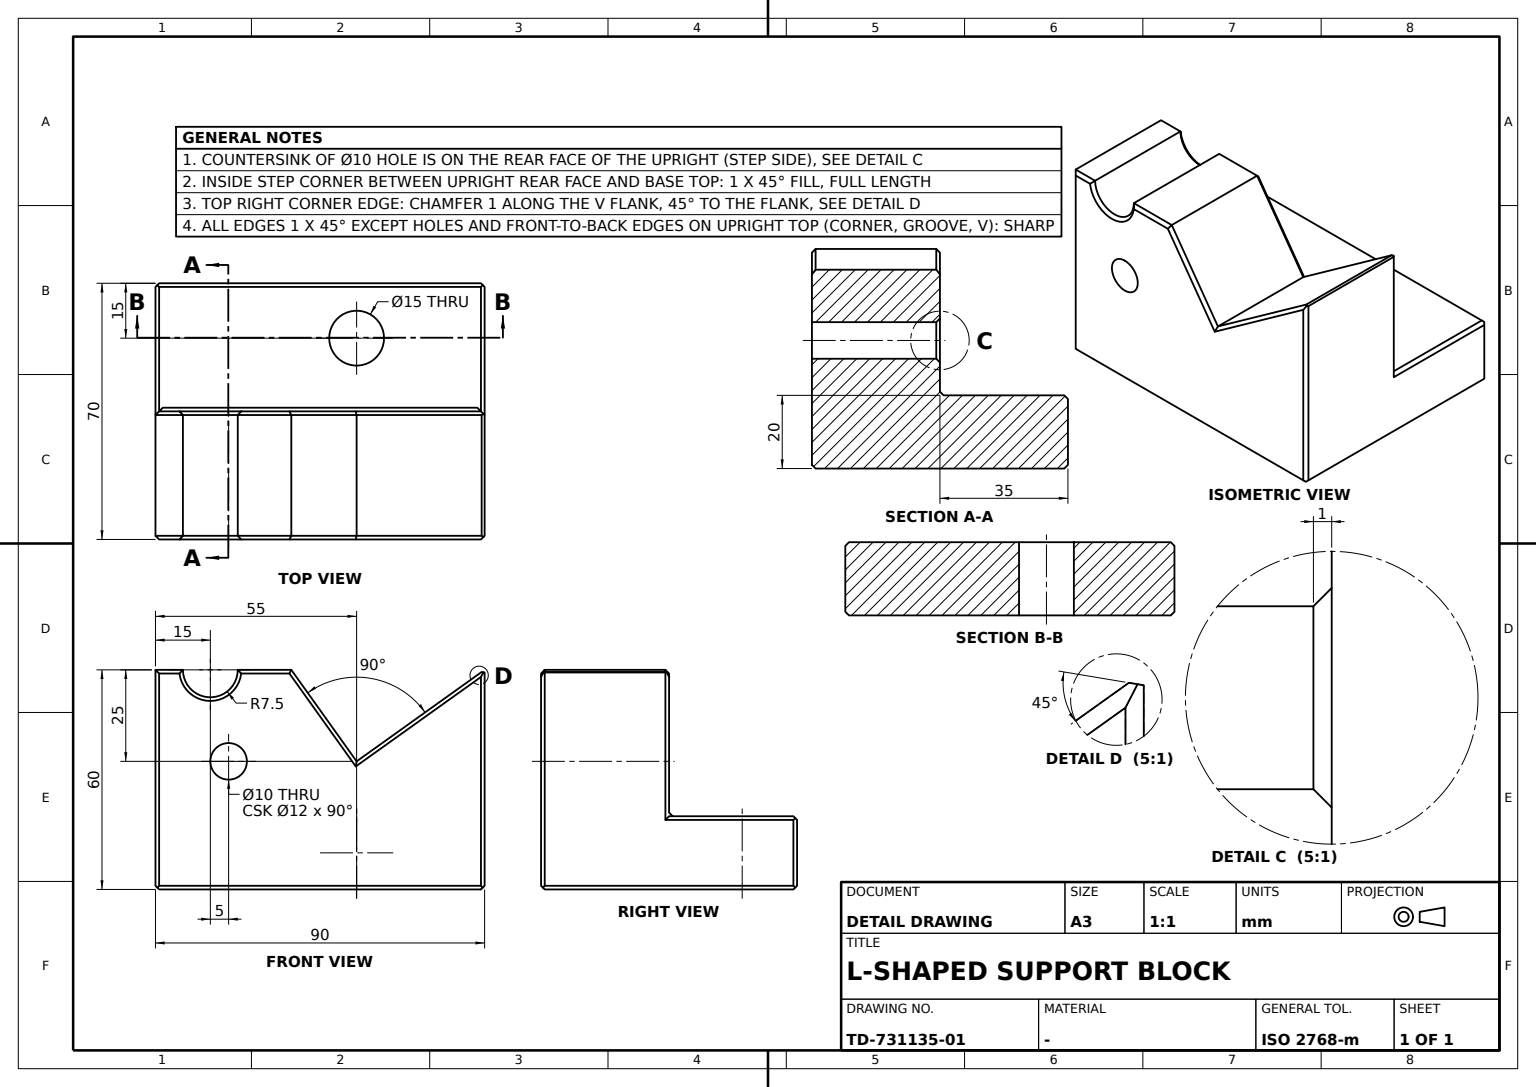
ISO-10303-21;
HEADER;
FILE_DESCRIPTION((''),'2;1');
FILE_NAME('','',(''),(''),'','','');
FILE_SCHEMA(('AUTOMOTIVE_DESIGN'));
ENDSEC;
DATA;
#1=APPLICATION_CONTEXT('');
#2=PRODUCT_CONTEXT('',#1,'mechanical');
#3=PRODUCT('','','',(#2));
#4=PRODUCT_DEFINITION_FORMATION('','',#3);
#5=PRODUCT_DEFINITION_CONTEXT('',#1,'design');
#6=PRODUCT_DEFINITION('','',#4,#5);
#7=PRODUCT_DEFINITION_SHAPE('','',#6);
#8=(LENGTH_UNIT()NAMED_UNIT(*)SI_UNIT(.MILLI.,.METRE.));
#9=(NAMED_UNIT(*)PLANE_ANGLE_UNIT()SI_UNIT($,.RADIAN.));
#10=(NAMED_UNIT(*)SI_UNIT($,.STERADIAN.)SOLID_ANGLE_UNIT());
#11=UNCERTAINTY_MEASURE_WITH_UNIT(LENGTH_MEASURE(0.005),#8,'distance_accuracy_value','');
#12=(GEOMETRIC_REPRESENTATION_CONTEXT(3)GLOBAL_UNCERTAINTY_ASSIGNED_CONTEXT((#11))GLOBAL_UNIT_ASSIGNED_CONTEXT((#8,#9,#10))REPRESENTATION_CONTEXT('',''));
#13=CARTESIAN_POINT('',(-0.813733,-16.5,-0.581238));
#14=VERTEX_POINT('',#13);
#15=CARTESIAN_POINT('',(-0.339767,-16.839767,-0.660233));
#16=VERTEX_POINT('',#15);
#17=CARTESIAN_POINT('',(8.804835,-23.395171,-2.184333));
#18=DIRECTION('',(0.805387266,-0.577350269,-0.134231211));
#19=VECTOR('',#18,1000.);
#20=LINE('',#17,#19);
#21=EDGE_CURVE('',#14,#16,#20,.T.);
#22=ORIENTED_EDGE('',*,*,#21,.F.);
#23=CARTESIAN_POINT('',(-35.,-16.5,-25.));
#24=VERTEX_POINT('',#23);
#25=CARTESIAN_POINT('',(16.018762,-16.5,11.441973));
#26=DIRECTION('',(-0.813733471,0.,-0.581238194));
#27=VECTOR('',#26,1000.);
#28=LINE('',#25,#27);
#29=EDGE_CURVE('',#14,#24,#28,.T.);
#30=ORIENTED_EDGE('',*,*,#29,.T.);
#31=CARTESIAN_POINT('',(-35.232495,-17.5,-26.394972));
#32=VERTEX_POINT('',#31);
#33=CARTESIAN_POINT('',(-39.420834,-35.514728,-51.525007));
#34=DIRECTION('',(-0.134231211,-0.577350269,-0.805387266));
#35=VECTOR('',#34,1000.);
#36=LINE('',#33,#35);
#37=EDGE_CURVE('',#24,#32,#36,.T.);
#38=ORIENTED_EDGE('',*,*,#37,.T.);
#39=CARTESIAN_POINT('',(-1.,-17.5,-1.943189));
#40=VERTEX_POINT('',#39);
#41=CARTESIAN_POINT('',(16.6,-17.5,10.628239));
#42=LINE('',#41,#27);
#43=EDGE_CURVE('',#40,#32,#42,.T.);
#44=ORIENTED_EDGE('',*,*,#43,.F.);
#45=CARTESIAN_POINT('',(6.622712,-9.877288,12.869182));
#46=DIRECTION('',(0.416089715,0.416089715,0.808541092));
#47=VECTOR('',#46,1000.);
#48=LINE('',#45,#47);
#49=EDGE_CURVE('',#40,#16,#48,.T.);
#50=ORIENTED_EDGE('',*,*,#49,.T.);
#51=EDGE_LOOP('',(#22,#30,#38,#44,#50));
#52=FACE_BOUND('',#51,.T.);
#53=DIRECTION('',(-0.410997468,-0.707106781,0.575396456));
#54=AXIS2_PLACEMENT_3D('',#25,#53,#26);
#55=PLANE('',#54);
#56=ADVANCED_FACE('',(#52),#55,.T.);
#57=CARTESIAN_POINT('',(0.,16.5,-41.));
#58=VERTEX_POINT('',#57);
#59=CARTESIAN_POINT('',(0.,51.5,-41.));
#60=VERTEX_POINT('',#59);
#61=CARTESIAN_POINT('',(0.,-31.5,-41.));
#62=DIRECTION('',(0.,1.,0.));
#63=VECTOR('',#62,1000.);
#64=LINE('',#61,#63);
#65=EDGE_CURVE('',#58,#60,#64,.T.);
#66=ORIENTED_EDGE('',*,*,#65,.F.);
#67=CARTESIAN_POINT('',(0.,16.5,-0.71686));
#68=VERTEX_POINT('',#67);
#69=CARTESIAN_POINT('',(0.,16.5,-72.));
#70=DIRECTION('',(0.,0.,-1.));
#71=VECTOR('',#70,1000.);
#72=LINE('',#69,#71);
#73=EDGE_CURVE('',#68,#58,#72,.T.);
#74=ORIENTED_EDGE('',*,*,#73,.F.);
#75=CARTESIAN_POINT('',(0.,-16.5,-0.71686));
#76=VERTEX_POINT('',#75);
#77=CARTESIAN_POINT('',(0.,0.,-0.71686));
#78=LINE('',#77,#63);
#79=EDGE_CURVE('',#76,#68,#78,.T.);
#80=ORIENTED_EDGE('',*,*,#79,.F.);
#81=CARTESIAN_POINT('',(0.,-16.5,-59.));
#82=VERTEX_POINT('',#81);
#83=CARTESIAN_POINT('',(0.,-16.5,0.));
#84=LINE('',#83,#71);
#85=EDGE_CURVE('',#76,#82,#84,.T.);
#86=ORIENTED_EDGE('',*,*,#85,.T.);
#87=CARTESIAN_POINT('',(0.,51.5,-59.));
#88=VERTEX_POINT('',#87);
#89=CARTESIAN_POINT('',(0.,0.,-59.));
#90=LINE('',#89,#63);
#91=EDGE_CURVE('',#82,#88,#90,.T.);
#92=ORIENTED_EDGE('',*,*,#91,.T.);
#93=CARTESIAN_POINT('',(0.,51.5,0.));
#94=DIRECTION('',(0.,0.,1.));
#95=VECTOR('',#94,1000.);
#96=LINE('',#93,#95);
#97=EDGE_CURVE('',#88,#60,#96,.T.);
#98=ORIENTED_EDGE('',*,*,#97,.T.);
#99=EDGE_LOOP('',(#66,#74,#80,#86,#92,#98));
#100=FACE_BOUND('',#99,.T.);
#101=CARTESIAN_POINT('',(0.,0.,0.));
#102=DIRECTION('',(1.,0.,0.));
#103=AXIS2_PLACEMENT_3D('',#101,#102,#62);
#104=PLANE('',#103);
#105=ADVANCED_FACE('',(#100),#104,.T.);
#106=CARTESIAN_POINT('',(-67.5,-16.5,0.));
#107=VERTEX_POINT('',#106);
#108=CARTESIAN_POINT('',(-66.559028,-17.5,-1.));
#109=VERTEX_POINT('',#108);
#110=CARTESIAN_POINT('',(-67.172962,-16.827038,-0.327038));
#111=CARTESIAN_POINT('',(-66.860357,-17.160866,-0.660866));
#112=B_SPLINE_CURVE_WITH_KNOTS('',3,(#106,#110,#111,#108),.UNSPECIFIED.,.F.,.F.,(4,4),(0.,0.001698655),.UNSPECIFIED.);
#113=EDGE_CURVE('',#107,#109,#112,.T.);
#114=ORIENTED_EDGE('',*,*,#113,.T.);
#115=CARTESIAN_POINT('',(-53.371761,-17.5,-1.));
#116=VERTEX_POINT('',#115);
#117=CARTESIAN_POINT('',(-106.6,-17.5,-1.));
#118=VECTOR('',#102,1000.);
#119=LINE('',#117,#118);
#120=EDGE_CURVE('',#109,#116,#119,.T.);
#121=ORIENTED_EDGE('',*,*,#120,.T.);
#122=CARTESIAN_POINT('',(-52.857143,-16.5,0.));
#123=VERTEX_POINT('',#122);
#124=CARTESIAN_POINT('',(-59.14141,-28.71152,-12.21152));
#125=DIRECTION('',(-0.341953402,-0.664480199,-0.664480199));
#126=VECTOR('',#125,1000.);
#127=LINE('',#124,#126);
#128=EDGE_CURVE('',#123,#116,#127,.T.);
#129=ORIENTED_EDGE('',*,*,#128,.F.);
#130=LINE('',#83,#118);
#131=EDGE_CURVE('',#107,#123,#130,.T.);
#132=ORIENTED_EDGE('',*,*,#131,.F.);
#133=EDGE_LOOP('',(#114,#121,#129,#132));
#134=FACE_BOUND('',#133,.T.);
#135=CARTESIAN_POINT('',(-106.6,-16.5,0.));
#136=DIRECTION('',(0.,0.707106781,-0.707106781));
#137=AXIS2_PLACEMENT_3D('',#135,#136,#102);
#138=PLANE('',#137);
#139=ADVANCED_FACE('',(#134),#138,.F.);
#140=CARTESIAN_POINT('',(-1.,17.5,-40.));
#141=VERTEX_POINT('',#140);
#142=CARTESIAN_POINT('',(9.666667,6.833333,-50.666667));
#143=DIRECTION('',(0.577350269,-0.577350269,-0.577350269));
#144=VECTOR('',#143,1000.);
#145=LINE('',#142,#144);
#146=EDGE_CURVE('',#141,#58,#145,.T.);
#147=ORIENTED_EDGE('',*,*,#146,.T.);
#148=ORIENTED_EDGE('',*,*,#65,.T.);
#149=CARTESIAN_POINT('',(-0.5,52.,-40.5));
#150=VERTEX_POINT('',#149);
#151=CARTESIAN_POINT('',(9.666667,41.833333,-50.666667));
#152=LINE('',#151,#144);
#153=EDGE_CURVE('',#150,#60,#152,.T.);
#154=ORIENTED_EDGE('',*,*,#153,.F.);
#155=CARTESIAN_POINT('',(-1.,51.5,-40.));
#156=VERTEX_POINT('',#155);
#157=CARTESIAN_POINT('',(-36.,16.5,-5.));
#158=DIRECTION('',(-0.577350269,-0.577350269,0.577350269));
#159=VECTOR('',#158,1000.);
#160=LINE('',#157,#159);
#161=EDGE_CURVE('',#150,#156,#160,.T.);
#162=ORIENTED_EDGE('',*,*,#161,.T.);
#163=CARTESIAN_POINT('',(-1.,-31.5,-40.));
#164=LINE('',#163,#63);
#165=EDGE_CURVE('',#141,#156,#164,.T.);
#166=ORIENTED_EDGE('',*,*,#165,.F.);
#167=EDGE_LOOP('',(#147,#148,#154,#162,#166));
#168=FACE_BOUND('',#167,.T.);
#169=DIRECTION('',(0.707106781,0.,0.707106781));
#170=AXIS2_PLACEMENT_3D('',#61,#169,#62);
#171=PLANE('',#170);
#172=ADVANCED_FACE('',(#168),#171,.T.);
#173=CARTESIAN_POINT('',(-90.,16.5,0.));
#174=VERTEX_POINT('',#173);
#175=CARTESIAN_POINT('',(-90.,16.5,-41.));
#176=VERTEX_POINT('',#175);
#177=LINE('',#173,#71);
#178=EDGE_CURVE('',#174,#176,#177,.T.);
#179=ORIENTED_EDGE('',*,*,#178,.F.);
#180=CARTESIAN_POINT('',(-89.,17.5,-1.));
#181=VERTEX_POINT('',#180);
#182=CARTESIAN_POINT('',(-65.333333,41.166667,-24.666667));
#183=DIRECTION('',(0.577350269,0.577350269,-0.577350269));
#184=VECTOR('',#183,1000.);
#185=LINE('',#182,#184);
#186=EDGE_CURVE('',#174,#181,#185,.T.);
#187=ORIENTED_EDGE('',*,*,#186,.T.);
#188=CARTESIAN_POINT('',(-89.,17.5,-39.));
#189=VERTEX_POINT('',#188);
#190=CARTESIAN_POINT('',(-89.,17.5,-40.));
#191=LINE('',#190,#95);
#192=EDGE_CURVE('',#189,#181,#191,.T.);
#193=ORIENTED_EDGE('',*,*,#192,.F.);
#194=CARTESIAN_POINT('',(-88.,18.5,-40.));
#195=VERTEX_POINT('',#194);
#196=CARTESIAN_POINT('',(-78.,28.5,-50.));
#197=LINE('',#196,#159);
#198=EDGE_CURVE('',#195,#189,#197,.T.);
#199=ORIENTED_EDGE('',*,*,#198,.F.);
#200=VERTEX_POINT('',#190);
#201=DIRECTION('',(0.707106781,0.707106781,0.));
#202=VECTOR('',#201,1000.);
#203=LINE('',#190,#202);
#204=EDGE_CURVE('',#200,#195,#203,.T.);
#205=ORIENTED_EDGE('',*,*,#204,.F.);
#206=CARTESIAN_POINT('',(-106.,0.5,-57.));
#207=DIRECTION('',(-0.577350269,-0.577350269,-0.577350269));
#208=VECTOR('',#207,1000.);
#209=LINE('',#206,#208);
#210=EDGE_CURVE('',#200,#176,#209,.T.);
#211=ORIENTED_EDGE('',*,*,#210,.T.);
#212=EDGE_LOOP('',(#179,#187,#193,#199,#205,#211));
#213=FACE_BOUND('',#212,.T.);
#214=CARTESIAN_POINT('',(-89.,17.5,-72.));
#215=DIRECTION('',(0.707106781,-0.707106781,0.));
#216=AXIS2_PLACEMENT_3D('',#214,#215,#94);
#217=PLANE('',#216);
#218=ADVANCED_FACE('',(#213),#217,.F.);
#219=CARTESIAN_POINT('',(-82.5,16.5,0.));
#220=VERTEX_POINT('',#219);
#221=CARTESIAN_POINT('',(-83.440972,17.5,-1.));
#222=VERTEX_POINT('',#221);
#223=CARTESIAN_POINT('',(-83.139643,17.160866,-0.660866));
#224=CARTESIAN_POINT('',(-82.827038,16.827038,-0.327038));
#225=B_SPLINE_CURVE_WITH_KNOTS('',3,(#221,#223,#224,#219),.UNSPECIFIED.,.F.,.F.,(4,4),(0.,0.001698655),.UNSPECIFIED.);
#226=EDGE_CURVE('',#220,#222,#225,.F.);
#227=ORIENTED_EDGE('',*,*,#226,.T.);
#228=CARTESIAN_POINT('',(0.,17.5,-1.));
#229=LINE('',#228,#118);
#230=EDGE_CURVE('',#181,#222,#229,.T.);
#231=ORIENTED_EDGE('',*,*,#230,.F.);
#232=ORIENTED_EDGE('',*,*,#186,.F.);
#233=CARTESIAN_POINT('',(-106.6,16.5,0.));
#234=LINE('',#233,#118);
#235=EDGE_CURVE('',#174,#220,#234,.T.);
#236=ORIENTED_EDGE('',*,*,#235,.T.);
#237=EDGE_LOOP('',(#227,#231,#232,#236));
#238=FACE_BOUND('',#237,.T.);
#239=CARTESIAN_POINT('',(-106.6,17.5,-1.));
#240=DIRECTION('',(0.,-0.707106781,-0.707106781));
#241=AXIS2_PLACEMENT_3D('',#239,#240,#102);
#242=PLANE('',#241);
#243=ADVANCED_FACE('',(#238),#242,.F.);
#244=CARTESIAN_POINT('',(-89.,51.5,-40.));
#245=VERTEX_POINT('',#244);
#246=CARTESIAN_POINT('',(-89.,-31.5,-40.));
#247=LINE('',#246,#63);
#248=EDGE_CURVE('',#200,#245,#247,.T.);
#249=ORIENTED_EDGE('',*,*,#248,.T.);
#250=CARTESIAN_POINT('',(-89.5,52.,-40.5));
#251=VERTEX_POINT('',#250);
#252=CARTESIAN_POINT('',(-96.,58.5,-47.));
#253=DIRECTION('',(0.577350269,-0.577350269,0.577350269));
#254=VECTOR('',#253,1000.);
#255=LINE('',#252,#254);
#256=EDGE_CURVE('',#251,#245,#255,.T.);
#257=ORIENTED_EDGE('',*,*,#256,.F.);
#258=CARTESIAN_POINT('',(-90.,51.5,-41.));
#259=VERTEX_POINT('',#258);
#260=CARTESIAN_POINT('',(-117.666667,23.833333,-68.666667));
#261=LINE('',#260,#208);
#262=EDGE_CURVE('',#251,#259,#261,.T.);
#263=ORIENTED_EDGE('',*,*,#262,.T.);
#264=CARTESIAN_POINT('',(-90.,0.,-41.));
#265=LINE('',#264,#63);
#266=EDGE_CURVE('',#176,#259,#265,.T.);
#267=ORIENTED_EDGE('',*,*,#266,.F.);
#268=ORIENTED_EDGE('',*,*,#210,.F.);
#269=EDGE_LOOP('',(#249,#257,#263,#267,#268));
#270=FACE_BOUND('',#269,.T.);
#271=CARTESIAN_POINT('',(-90.,-31.5,-41.));
#272=DIRECTION('',(0.707106781,0.,-0.707106781));
#273=AXIS2_PLACEMENT_3D('',#271,#272,#62);
#274=PLANE('',#273);
#275=ADVANCED_FACE('',(#270),#274,.F.);
#276=CARTESIAN_POINT('',(-90.,-16.5,-59.));
#277=VERTEX_POINT('',#276);
#278=CARTESIAN_POINT('',(-90.,-16.5,0.));
#279=VERTEX_POINT('',#278);
#280=LINE('',#278,#95);
#281=EDGE_CURVE('',#277,#279,#280,.T.);
#282=ORIENTED_EDGE('',*,*,#281,.T.);
#283=CARTESIAN_POINT('',(-90.,17.5,0.));
#284=DIRECTION('',(0.,-1.,0.));
#285=VECTOR('',#284,1000.);
#286=LINE('',#283,#285);
#287=EDGE_CURVE('',#174,#279,#286,.T.);
#288=ORIENTED_EDGE('',*,*,#287,.F.);
#289=ORIENTED_EDGE('',*,*,#178,.T.);
#290=ORIENTED_EDGE('',*,*,#266,.T.);
#291=CARTESIAN_POINT('',(-90.,51.5,-59.));
#292=VERTEX_POINT('',#291);
#293=CARTESIAN_POINT('',(-90.,51.5,0.));
#294=LINE('',#293,#71);
#295=EDGE_CURVE('',#259,#292,#294,.T.);
#296=ORIENTED_EDGE('',*,*,#295,.T.);
#297=CARTESIAN_POINT('',(-90.,0.,-59.));
#298=LINE('',#297,#285);
#299=EDGE_CURVE('',#292,#277,#298,.T.);
#300=ORIENTED_EDGE('',*,*,#299,.T.);
#301=EDGE_LOOP('',(#282,#288,#289,#290,#296,#300));
#302=FACE_BOUND('',#301,.T.);
#303=CARTESIAN_POINT('',(-90.,0.,0.));
#304=AXIS2_PLACEMENT_3D('',#303,#102,#62);
#305=PLANE('',#304);
#306=ADVANCED_FACE('',(#302),#305,.F.);
#307=CARTESIAN_POINT('',(-35.,16.5,-25.));
#308=VERTEX_POINT('',#307);
#309=CARTESIAN_POINT('',(-35.,17.5,-25.));
#310=LINE('',#309,#285);
#311=EDGE_CURVE('',#308,#24,#310,.T.);
#312=ORIENTED_EDGE('',*,*,#311,.F.);
#313=CARTESIAN_POINT('',(-52.857143,16.5,0.));
#314=VERTEX_POINT('',#313);
#315=DIRECTION('',(-0.581238194,0.,0.813733471));
#316=VECTOR('',#315,1000.);
#317=LINE('',#307,#316);
#318=EDGE_CURVE('',#308,#314,#317,.T.);
#319=ORIENTED_EDGE('',*,*,#318,.T.);
#320=CARTESIAN_POINT('',(-52.857143,17.5,0.));
#321=LINE('',#320,#285);
#322=EDGE_CURVE('',#314,#123,#321,.T.);
#323=ORIENTED_EDGE('',*,*,#322,.T.);
#324=CARTESIAN_POINT('',(-1.843742,-16.5,-71.418762));
#325=LINE('',#324,#316);
#326=EDGE_CURVE('',#24,#123,#325,.T.);
#327=ORIENTED_EDGE('',*,*,#326,.F.);
#328=EDGE_LOOP('',(#312,#319,#323,#327));
#329=FACE_BOUND('',#328,.T.);
#330=DIRECTION('',(0.813733471,0.,0.581238194));
#331=AXIS2_PLACEMENT_3D('',#309,#330,#315);
#332=PLANE('',#331);
#333=ADVANCED_FACE('',(#329),#332,.T.);
#334=CARTESIAN_POINT('',(-35.232495,17.5,-26.394972));
#335=VERTEX_POINT('',#334);
#336=CARTESIAN_POINT('',(-37.175831,25.858604,-38.054988));
#337=DIRECTION('',(0.134231211,-0.577350269,0.805387266));
#338=VECTOR('',#337,1000.);
#339=LINE('',#336,#338);
#340=EDGE_CURVE('',#335,#308,#339,.T.);
#341=ORIENTED_EDGE('',*,*,#340,.F.);
#342=CARTESIAN_POINT('',(-53.371761,17.5,-1.));
#343=VERTEX_POINT('',#342);
#344=CARTESIAN_POINT('',(-16.894815,17.5,-52.067725));
#345=LINE('',#344,#316);
#346=EDGE_CURVE('',#335,#343,#345,.T.);
#347=ORIENTED_EDGE('',*,*,#346,.T.);
#348=CARTESIAN_POINT('',(-59.595852,29.594588,-13.094588));
#349=DIRECTION('',(0.341953402,-0.664480199,0.664480199));
#350=VECTOR('',#349,1000.);
#351=LINE('',#348,#350);
#352=EDGE_CURVE('',#343,#314,#351,.T.);
#353=ORIENTED_EDGE('',*,*,#352,.T.);
#354=ORIENTED_EDGE('',*,*,#318,.F.);
#355=EDGE_LOOP('',(#341,#347,#353,#354));
#356=FACE_BOUND('',#355,.T.);
#357=CARTESIAN_POINT('',(-20.657475,17.5,-46.8));
#358=DIRECTION('',(0.575396456,0.707106781,0.410997468));
#359=AXIS2_PLACEMENT_3D('',#357,#358,#315);
#360=PLANE('',#359);
#361=ADVANCED_FACE('',(#356),#360,.T.);
#362=ORIENTED_EDGE('',*,*,#299,.F.);
#363=CARTESIAN_POINT('',(-89.5,52.,-59.5));
#364=VERTEX_POINT('',#363);
#365=CARTESIAN_POINT('',(-113.666667,27.833333,-35.333333));
#366=LINE('',#365,#159);
#367=EDGE_CURVE('',#364,#292,#366,.T.);
#368=ORIENTED_EDGE('',*,*,#367,.F.);
#369=CARTESIAN_POINT('',(-89.,51.5,-60.));
#370=VERTEX_POINT('',#369);
#371=CARTESIAN_POINT('',(-94.266667,56.766667,-54.733333));
#372=LINE('',#371,#144);
#373=EDGE_CURVE('',#364,#370,#372,.T.);
#374=ORIENTED_EDGE('',*,*,#373,.T.);
#375=CARTESIAN_POINT('',(-89.,-16.5,-60.));
#376=VERTEX_POINT('',#375);
#377=CARTESIAN_POINT('',(-89.,65.3,-60.));
#378=LINE('',#377,#285);
#379=EDGE_CURVE('',#370,#376,#378,.T.);
#380=ORIENTED_EDGE('',*,*,#379,.T.);
#381=CARTESIAN_POINT('',(-89.5,-17.,-59.5));
#382=VERTEX_POINT('',#381);
#383=CARTESIAN_POINT('',(-53.8,18.7,-95.2));
#384=LINE('',#383,#184);
#385=EDGE_CURVE('',#382,#376,#384,.T.);
#386=ORIENTED_EDGE('',*,*,#385,.F.);
#387=CARTESIAN_POINT('',(-85.666667,-20.833333,-63.333333));
#388=LINE('',#387,#144);
#389=EDGE_CURVE('',#277,#382,#388,.T.);
#390=ORIENTED_EDGE('',*,*,#389,.F.);
#391=EDGE_LOOP('',(#362,#368,#374,#380,#386,#390));
#392=FACE_BOUND('',#391,.T.);
#393=CARTESIAN_POINT('',(-90.,65.3,-59.));
#394=AXIS2_PLACEMENT_3D('',#393,#169,#284);
#395=PLANE('',#394);
#396=ADVANCED_FACE('',(#392),#395,.F.);
#397=CARTESIAN_POINT('',(-7.71107,-24.21107,0.568318));
#398=DIRECTION('',(-0.702246883,-0.702246883,0.117041147));
#399=VECTOR('',#398,1000.);
#400=LINE('',#397,#399);
#401=EDGE_CURVE('',#76,#16,#400,.T.);
#402=ORIENTED_EDGE('',*,*,#401,.T.);
#403=ORIENTED_EDGE('',*,*,#49,.F.);
#404=CARTESIAN_POINT('',(-1.,-17.5,-59.));
#405=VERTEX_POINT('',#404);
#406=CARTESIAN_POINT('',(-1.,-17.5,0.));
#407=LINE('',#406,#71);
#408=EDGE_CURVE('',#40,#405,#407,.T.);
#409=ORIENTED_EDGE('',*,*,#408,.T.);
#410=CARTESIAN_POINT('',(-0.5,-17.,-59.5));
#411=VERTEX_POINT('',#410);
#412=CARTESIAN_POINT('',(-24.666667,-41.166667,-35.333333));
#413=LINE('',#412,#159);
#414=EDGE_CURVE('',#411,#405,#413,.T.);
#415=ORIENTED_EDGE('',*,*,#414,.F.);
#416=CARTESIAN_POINT('',(23.,6.5,-36.));
#417=DIRECTION('',(0.577350269,0.577350269,0.577350269));
#418=VECTOR('',#417,1000.);
#419=LINE('',#416,#418);
#420=EDGE_CURVE('',#411,#82,#419,.T.);
#421=ORIENTED_EDGE('',*,*,#420,.T.);
#422=ORIENTED_EDGE('',*,*,#85,.F.);
#423=EDGE_LOOP('',(#402,#403,#409,#415,#421,#422));
#424=FACE_BOUND('',#423,.T.);
#425=CARTESIAN_POINT('',(-1.,-17.5,12.));
#426=AXIS2_PLACEMENT_3D('',#425,#215,#70);
#427=PLANE('',#426);
#428=ADVANCED_FACE('',(#424),#427,.T.);
#429=CARTESIAN_POINT('',(-70.,-17.5,-20.));
#430=VERTEX_POINT('',#429);
#431=CARTESIAN_POINT('',(-70.,-17.5,-25.));
#432=AXIS2_PLACEMENT_3D('',#431,#62,#94);
#433=CIRCLE('',#432,5.);
#434=EDGE_CURVE('',#430,#430,#433,.T.);
#435=ORIENTED_EDGE('',*,*,#434,.T.);
#436=EDGE_LOOP('',(#435));
#437=FACE_BOUND('',#436,.T.);
#438=ORIENTED_EDGE('',*,*,#408,.F.);
#439=ORIENTED_EDGE('',*,*,#43,.T.);
#440=CARTESIAN_POINT('',(-2.657475,-17.5,-72.));
#441=LINE('',#440,#316);
#442=EDGE_CURVE('',#32,#116,#441,.T.);
#443=ORIENTED_EDGE('',*,*,#442,.T.);
#444=ORIENTED_EDGE('',*,*,#120,.F.);
#445=CARTESIAN_POINT('',(-83.440972,-17.5,-1.));
#446=VERTEX_POINT('',#445);
#447=CARTESIAN_POINT('',(-75.,-17.5,0.));
#448=AXIS2_PLACEMENT_3D('',#447,#62,#94);
#449=CIRCLE('',#448,8.5);
#450=EDGE_CURVE('',#109,#446,#449,.T.);
#451=ORIENTED_EDGE('',*,*,#450,.T.);
#452=CARTESIAN_POINT('',(-89.,-17.5,-1.));
#453=VERTEX_POINT('',#452);
#454=EDGE_CURVE('',#453,#446,#119,.T.);
#455=ORIENTED_EDGE('',*,*,#454,.F.);
#456=CARTESIAN_POINT('',(-89.,-17.5,-59.));
#457=VERTEX_POINT('',#456);
#458=CARTESIAN_POINT('',(-89.,-17.5,-72.));
#459=LINE('',#458,#95);
#460=EDGE_CURVE('',#457,#453,#459,.T.);
#461=ORIENTED_EDGE('',*,*,#460,.F.);
#462=CARTESIAN_POINT('',(16.6,-17.5,-59.));
#463=DIRECTION('',(-1.,0.,0.));
#464=VECTOR('',#463,1000.);
#465=LINE('',#462,#464);
#466=EDGE_CURVE('',#405,#457,#465,.T.);
#467=ORIENTED_EDGE('',*,*,#466,.F.);
#468=EDGE_LOOP('',(#438,#439,#443,#444,#451,#455,#461,#467));
#469=FACE_BOUND('',#468,.T.);
#470=CARTESIAN_POINT('',(0.,-17.5,0.));
#471=AXIS2_PLACEMENT_3D('',#470,#62,#70);
#472=PLANE('',#471);
#473=ADVANCED_FACE('',(#437,#469),#472,.F.);
#474=ORIENTED_EDGE('',*,*,#460,.T.);
#475=CARTESIAN_POINT('',(-95.533333,-10.966667,5.533333));
#476=LINE('',#475,#144);
#477=EDGE_CURVE('',#279,#453,#476,.T.);
#478=ORIENTED_EDGE('',*,*,#477,.F.);
#479=ORIENTED_EDGE('',*,*,#281,.F.);
#480=ORIENTED_EDGE('',*,*,#389,.T.);
#481=CARTESIAN_POINT('',(-94.,-12.5,-64.));
#482=LINE('',#481,#254);
#483=EDGE_CURVE('',#382,#457,#482,.T.);
#484=ORIENTED_EDGE('',*,*,#483,.T.);
#485=EDGE_LOOP('',(#474,#478,#479,#480,#484));
#486=FACE_BOUND('',#485,.T.);
#487=CARTESIAN_POINT('',(-90.,-16.5,-72.));
#488=AXIS2_PLACEMENT_3D('',#487,#201,#94);
#489=PLANE('',#488);
#490=ADVANCED_FACE('',(#486),#489,.F.);
#491=CARTESIAN_POINT('',(-2.,18.5,-40.));
#492=VERTEX_POINT('',#491);
#493=CARTESIAN_POINT('',(0.,18.5,-40.));
#494=LINE('',#493,#118);
#495=EDGE_CURVE('',#195,#492,#494,.T.);
#496=ORIENTED_EDGE('',*,*,#495,.F.);
#497=ORIENTED_EDGE('',*,*,#198,.T.);
#498=CARTESIAN_POINT('',(-1.,17.5,-39.));
#499=VERTEX_POINT('',#498);
#500=CARTESIAN_POINT('',(-108.,17.5,-39.));
#501=LINE('',#500,#118);
#502=EDGE_CURVE('',#189,#499,#501,.T.);
#503=ORIENTED_EDGE('',*,*,#502,.T.);
#504=CARTESIAN_POINT('',(-12.,28.5,-50.));
#505=LINE('',#504,#254);
#506=EDGE_CURVE('',#492,#499,#505,.T.);
#507=ORIENTED_EDGE('',*,*,#506,.F.);
#508=EDGE_LOOP('',(#496,#497,#503,#507));
#509=FACE_BOUND('',#508,.T.);
#510=DIRECTION('',(0.,0.707106781,0.707106781));
#511=AXIS2_PLACEMENT_3D('',#500,#510,#102);
#512=PLANE('',#511);
#513=ADVANCED_FACE('',(#509),#512,.T.);
#514=ORIENTED_EDGE('',*,*,#434,.F.);
#515=EDGE_LOOP('',(#514));
#516=FACE_BOUND('',#515,.T.);
#517=CARTESIAN_POINT('',(-70.,16.5,-20.));
#518=VERTEX_POINT('',#517);
#519=CARTESIAN_POINT('',(-70.,16.5,-25.));
#520=AXIS2_PLACEMENT_3D('',#519,#62,#94);
#521=CIRCLE('',#520,5.);
#522=EDGE_CURVE('',#518,#518,#521,.F.);
#523=ORIENTED_EDGE('',*,*,#522,.F.);
#524=EDGE_LOOP('',(#523));
#525=FACE_BOUND('',#524,.T.);
#526=CARTESIAN_POINT('',(-70.,-0.66,-25.));
#527=AXIS2_PLACEMENT_3D('',#526,#62,#463);
#528=CYLINDRICAL_SURFACE('',#527,5.);
#529=ADVANCED_FACE('',(#516,#525),#528,.F.);
#530=ORIENTED_EDGE('',*,*,#352,.F.);
#531=CARTESIAN_POINT('',(-66.559028,17.5,-1.));
#532=VERTEX_POINT('',#531);
#533=EDGE_CURVE('',#532,#343,#229,.T.);
#534=ORIENTED_EDGE('',*,*,#533,.F.);
#535=CARTESIAN_POINT('',(-67.5,16.5,0.));
#536=VERTEX_POINT('',#535);
#537=CARTESIAN_POINT('',(-66.860357,17.160866,-0.660866));
#538=CARTESIAN_POINT('',(-67.172962,16.827038,-0.327038));
#539=B_SPLINE_CURVE_WITH_KNOTS('',3,(#531,#537,#538,#535),.UNSPECIFIED.,.F.,.F.,(4,4),(0.,0.001698655),.UNSPECIFIED.);
#540=EDGE_CURVE('',#532,#536,#539,.T.);
#541=ORIENTED_EDGE('',*,*,#540,.T.);
#542=EDGE_CURVE('',#536,#314,#234,.T.);
#543=ORIENTED_EDGE('',*,*,#542,.T.);
#544=EDGE_LOOP('',(#530,#534,#541,#543));
#545=FACE_BOUND('',#544,.T.);
#546=ADVANCED_FACE('',(#545),#242,.F.);
#547=CARTESIAN_POINT('',(-42.5,37.5,-40.));
#548=VERTEX_POINT('',#547);
#549=CARTESIAN_POINT('',(-35.,37.5,-40.));
#550=AXIS2_PLACEMENT_3D('',#549,#70,#463);
#551=CIRCLE('',#550,7.5);
#552=EDGE_CURVE('',#548,#548,#551,.F.);
#553=ORIENTED_EDGE('',*,*,#552,.F.);
#554=EDGE_LOOP('',(#553));
#555=FACE_BOUND('',#554,.T.);
#556=CARTESIAN_POINT('',(-108.,51.5,-40.));
#557=LINE('',#556,#118);
#558=EDGE_CURVE('',#245,#156,#557,.T.);
#559=ORIENTED_EDGE('',*,*,#558,.F.);
#560=ORIENTED_EDGE('',*,*,#248,.F.);
#561=ORIENTED_EDGE('',*,*,#204,.T.);
#562=ORIENTED_EDGE('',*,*,#495,.T.);
#563=DIRECTION('',(-0.707106781,0.707106781,0.));
#564=VECTOR('',#563,1000.);
#565=LINE('',#140,#564);
#566=EDGE_CURVE('',#141,#492,#565,.T.);
#567=ORIENTED_EDGE('',*,*,#566,.F.);
#568=ORIENTED_EDGE('',*,*,#165,.T.);
#569=EDGE_LOOP('',(#559,#560,#561,#562,#567,#568));
#570=FACE_BOUND('',#569,.T.);
#571=CARTESIAN_POINT('',(0.,52.5,-40.));
#572=AXIS2_PLACEMENT_3D('',#571,#70,#284);
#573=PLANE('',#572);
#574=ADVANCED_FACE('',(#555,#570),#573,.F.);
#575=CARTESIAN_POINT('',(-0.5,52.,-59.5));
#576=VERTEX_POINT('',#575);
#577=CARTESIAN_POINT('',(27.,24.5,-32.));
#578=LINE('',#577,#254);
#579=EDGE_CURVE('',#576,#88,#578,.T.);
#580=ORIENTED_EDGE('',*,*,#579,.F.);
#581=CARTESIAN_POINT('',(-1.,52.5,-59.));
#582=VERTEX_POINT('',#581);
#583=CARTESIAN_POINT('',(-35.933333,87.433333,-24.066667));
#584=DIRECTION('',(-0.577350269,0.577350269,0.577350269));
#585=VECTOR('',#584,1000.);
#586=LINE('',#583,#585);
#587=EDGE_CURVE('',#576,#582,#586,.T.);
#588=ORIENTED_EDGE('',*,*,#587,.T.);
#589=CARTESIAN_POINT('',(-1.,52.5,-41.));
#590=VERTEX_POINT('',#589);
#591=CARTESIAN_POINT('',(-1.,52.5,-60.));
#592=LINE('',#591,#95);
#593=EDGE_CURVE('',#582,#590,#592,.T.);
#594=ORIENTED_EDGE('',*,*,#593,.T.);
#595=CARTESIAN_POINT('',(-11.333333,62.833333,-51.333333));
#596=DIRECTION('',(-0.577350269,0.577350269,-0.577350269));
#597=VECTOR('',#596,1000.);
#598=LINE('',#595,#597);
#599=EDGE_CURVE('',#150,#590,#598,.T.);
#600=ORIENTED_EDGE('',*,*,#599,.F.);
#601=ORIENTED_EDGE('',*,*,#153,.T.);
#602=ORIENTED_EDGE('',*,*,#97,.F.);
#603=EDGE_LOOP('',(#580,#588,#594,#600,#601,#602));
#604=FACE_BOUND('',#603,.T.);
#605=CARTESIAN_POINT('',(-1.,52.5,-72.));
#606=AXIS2_PLACEMENT_3D('',#605,#201,#94);
#607=PLANE('',#606);
#608=ADVANCED_FACE('',(#604),#607,.T.);
#609=ORIENTED_EDGE('',*,*,#414,.T.);
#610=ORIENTED_EDGE('',*,*,#466,.T.);
#611=ORIENTED_EDGE('',*,*,#483,.F.);
#612=ORIENTED_EDGE('',*,*,#385,.T.);
#613=CARTESIAN_POINT('',(-1.,-16.5,-60.));
#614=VERTEX_POINT('',#613);
#615=CARTESIAN_POINT('',(0.,-16.5,-60.));
#616=LINE('',#615,#464);
#617=EDGE_CURVE('',#614,#376,#616,.T.);
#618=ORIENTED_EDGE('',*,*,#617,.F.);
#619=CARTESIAN_POINT('',(4.866667,-22.366667,-54.133333));
#620=LINE('',#619,#597);
#621=EDGE_CURVE('',#411,#614,#620,.T.);
#622=ORIENTED_EDGE('',*,*,#621,.F.);
#623=EDGE_LOOP('',(#609,#610,#611,#612,#618,#622));
#624=FACE_BOUND('',#623,.T.);
#625=CARTESIAN_POINT('',(16.6,-16.5,-60.));
#626=AXIS2_PLACEMENT_3D('',#625,#510,#463);
#627=PLANE('',#626);
#628=ADVANCED_FACE('',(#624),#627,.F.);
#629=ORIENTED_EDGE('',*,*,#340,.T.);
#630=CARTESIAN_POINT('',(-0.813733,16.5,-0.581238));
#631=VERTEX_POINT('',#630);
#632=CARTESIAN_POINT('',(0.,16.5,0.));
#633=LINE('',#632,#27);
#634=EDGE_CURVE('',#631,#308,#633,.T.);
#635=ORIENTED_EDGE('',*,*,#634,.F.);
#636=CARTESIAN_POINT('',(-0.339767,16.839767,-0.660233));
#637=VERTEX_POINT('',#636);
#638=CARTESIAN_POINT('',(-23.040282,0.566667,3.123187));
#639=DIRECTION('',(0.805387266,0.577350269,-0.134231211));
#640=VECTOR('',#639,1000.);
#641=LINE('',#638,#640);
#642=EDGE_CURVE('',#631,#637,#641,.T.);
#643=ORIENTED_EDGE('',*,*,#642,.T.);
#644=CARTESIAN_POINT('',(-1.,17.5,-1.943189));
#645=VERTEX_POINT('',#644);
#646=CARTESIAN_POINT('',(4.639441,11.860559,9.015313));
#647=DIRECTION('',(-0.416089715,0.416089715,-0.808541092));
#648=VECTOR('',#647,1000.);
#649=LINE('',#646,#648);
#650=EDGE_CURVE('',#637,#645,#649,.T.);
#651=ORIENTED_EDGE('',*,*,#650,.T.);
#652=CARTESIAN_POINT('',(-18.337681,17.5,-14.327247));
#653=LINE('',#652,#27);
#654=EDGE_CURVE('',#645,#335,#653,.T.);
#655=ORIENTED_EDGE('',*,*,#654,.T.);
#656=EDGE_LOOP('',(#629,#635,#643,#651,#655));
#657=FACE_BOUND('',#656,.T.);
#658=CARTESIAN_POINT('',(12.640465,17.5,7.8));
#659=DIRECTION('',(-0.410997468,0.707106781,0.575396456));
#660=AXIS2_PLACEMENT_3D('',#658,#659,#26);
#661=PLANE('',#660);
#662=ADVANCED_FACE('',(#657),#661,.T.);
#663=CARTESIAN_POINT('',(-1.,51.5,-60.));
#664=VERTEX_POINT('',#663);
#665=CARTESIAN_POINT('',(-1.,-17.5,-60.));
#666=LINE('',#665,#63);
#667=EDGE_CURVE('',#614,#664,#666,.T.);
#668=ORIENTED_EDGE('',*,*,#667,.F.);
#669=ORIENTED_EDGE('',*,*,#617,.T.);
#670=ORIENTED_EDGE('',*,*,#379,.F.);
#671=CARTESIAN_POINT('',(0.,51.5,-60.));
#672=LINE('',#671,#118);
#673=EDGE_CURVE('',#370,#664,#672,.T.);
#674=ORIENTED_EDGE('',*,*,#673,.T.);
#675=EDGE_LOOP('',(#668,#669,#670,#674));
#676=FACE_BOUND('',#675,.T.);
#677=CARTESIAN_POINT('',(-27.5,37.5,-60.));
#678=VERTEX_POINT('',#677);
#679=CARTESIAN_POINT('',(-35.,37.5,-60.));
#680=AXIS2_PLACEMENT_3D('',#679,#94,#102);
#681=CIRCLE('',#680,7.5);
#682=EDGE_CURVE('',#678,#678,#681,.T.);
#683=ORIENTED_EDGE('',*,*,#682,.T.);
#684=EDGE_LOOP('',(#683));
#685=FACE_BOUND('',#684,.T.);
#686=CARTESIAN_POINT('',(0.,-17.5,-60.));
#687=AXIS2_PLACEMENT_3D('',#686,#94,#62);
#688=PLANE('',#687);
#689=ADVANCED_FACE('',(#676,#685),#688,.F.);
#690=ORIENTED_EDGE('',*,*,#682,.F.);
#691=EDGE_LOOP('',(#690));
#692=FACE_BOUND('',#691,.T.);
#693=ORIENTED_EDGE('',*,*,#552,.T.);
#694=EDGE_LOOP('',(#693));
#695=FACE_BOUND('',#694,.T.);
#696=CARTESIAN_POINT('',(-35.,37.5,-85.));
#697=AXIS2_PLACEMENT_3D('',#696,#94,#102);
#698=CYLINDRICAL_SURFACE('',#697,7.5);
#699=ADVANCED_FACE('',(#692,#695),#698,.F.);
#700=ORIENTED_EDGE('',*,*,#21,.T.);
#701=ORIENTED_EDGE('',*,*,#401,.F.);
#702=ORIENTED_EDGE('',*,*,#79,.T.);
#703=CARTESIAN_POINT('',(4.872587,11.627413,-1.528958));
#704=DIRECTION('',(-0.702246883,0.702246883,0.117041147));
#705=VECTOR('',#704,1000.);
#706=LINE('',#703,#705);
#707=EDGE_CURVE('',#68,#637,#706,.T.);
#708=ORIENTED_EDGE('',*,*,#707,.T.);
#709=ORIENTED_EDGE('',*,*,#642,.F.);
#710=CARTESIAN_POINT('',(-0.813733,-31.3,-0.581238));
#711=LINE('',#710,#63);
#712=EDGE_CURVE('',#14,#631,#711,.T.);
#713=ORIENTED_EDGE('',*,*,#712,.F.);
#714=EDGE_LOOP('',(#700,#701,#702,#708,#709,#713));
#715=FACE_BOUND('',#714,.T.);
#716=DIRECTION('',(-0.164398987,0.,-0.986393924));
#717=AXIS2_PLACEMENT_3D('',#710,#716,#62);
#718=PLANE('',#717);
#719=ADVANCED_FACE('',(#715),#718,.F.);
#720=CARTESIAN_POINT('',(-28.666667,23.833333,-87.666667));
#721=LINE('',#720,#208);
#722=EDGE_CURVE('',#576,#664,#721,.T.);
#723=ORIENTED_EDGE('',*,*,#722,.F.);
#724=ORIENTED_EDGE('',*,*,#579,.T.);
#725=ORIENTED_EDGE('',*,*,#91,.F.);
#726=ORIENTED_EDGE('',*,*,#420,.F.);
#727=ORIENTED_EDGE('',*,*,#621,.T.);
#728=ORIENTED_EDGE('',*,*,#667,.T.);
#729=EDGE_LOOP('',(#723,#724,#725,#726,#727,#728));
#730=FACE_BOUND('',#729,.T.);
#731=CARTESIAN_POINT('',(-1.,-31.5,-60.));
#732=AXIS2_PLACEMENT_3D('',#731,#272,#62);
#733=PLANE('',#732);
#734=ADVANCED_FACE('',(#730),#733,.T.);
#735=CARTESIAN_POINT('',(-75.,16.5,0.));
#736=AXIS2_PLACEMENT_3D('',#735,#62,#94);
#737=CIRCLE('',#736,7.5);
#738=EDGE_CURVE('',#220,#536,#737,.F.);
#739=ORIENTED_EDGE('',*,*,#738,.F.);
#740=CARTESIAN_POINT('',(-82.5,-16.5,0.));
#741=VERTEX_POINT('',#740);
#742=LINE('',#219,#63);
#743=EDGE_CURVE('',#741,#220,#742,.T.);
#744=ORIENTED_EDGE('',*,*,#743,.F.);
#745=CARTESIAN_POINT('',(-75.,-16.5,0.));
#746=AXIS2_PLACEMENT_3D('',#745,#284,#70);
#747=CIRCLE('',#746,7.5);
#748=EDGE_CURVE('',#107,#741,#747,.F.);
#749=ORIENTED_EDGE('',*,*,#748,.F.);
#750=LINE('',#535,#63);
#751=EDGE_CURVE('',#536,#107,#750,.F.);
#752=ORIENTED_EDGE('',*,*,#751,.F.);
#753=EDGE_LOOP('',(#739,#744,#749,#752));
#754=FACE_BOUND('',#753,.T.);
#755=CARTESIAN_POINT('',(-75.,-0.66,0.));
#756=AXIS2_PLACEMENT_3D('',#755,#62,#463);
#757=CYLINDRICAL_SURFACE('',#756,7.5);
#758=ADVANCED_FACE('',(#754),#757,.F.);
#759=ORIENTED_EDGE('',*,*,#128,.T.);
#760=ORIENTED_EDGE('',*,*,#442,.F.);
#761=ORIENTED_EDGE('',*,*,#37,.F.);
#762=ORIENTED_EDGE('',*,*,#326,.T.);
#763=EDGE_LOOP('',(#759,#760,#761,#762));
#764=FACE_BOUND('',#763,.T.);
#765=DIRECTION('',(0.575396456,-0.707106781,0.410997468));
#766=AXIS2_PLACEMENT_3D('',#324,#765,#315);
#767=PLANE('',#766);
#768=ADVANCED_FACE('',(#764),#767,.T.);
#769=CARTESIAN_POINT('',(-70.,17.5,-31.));
#770=VERTEX_POINT('',#769);
#771=CARTESIAN_POINT('',(-70.,17.5,-25.));
#772=AXIS2_PLACEMENT_3D('',#771,#284,#70);
#773=CIRCLE('',#772,6.);
#774=EDGE_CURVE('',#770,#770,#773,.T.);
#775=ORIENTED_EDGE('',*,*,#774,.F.);
#776=EDGE_LOOP('',(#775));
#777=FACE_BOUND('',#776,.T.);
#778=ORIENTED_EDGE('',*,*,#522,.T.);
#779=EDGE_LOOP('',(#778));
#780=FACE_BOUND('',#779,.T.);
#781=CARTESIAN_POINT('',(-70.,11.5,-25.));
#782=DIRECTION('',(-0.865680914,0.,0.5005962));
#783=AXIS2_PLACEMENT_3D('',#781,#62,#782);
#784=CONICAL_SURFACE('',#783,0.,0.785398163);
#785=ADVANCED_FACE('',(#777,#780),#784,.F.);
#786=ORIENTED_EDGE('',*,*,#650,.F.);
#787=ORIENTED_EDGE('',*,*,#707,.F.);
#788=ORIENTED_EDGE('',*,*,#73,.T.);
#789=ORIENTED_EDGE('',*,*,#146,.F.);
#790=ORIENTED_EDGE('',*,*,#566,.T.);
#791=ORIENTED_EDGE('',*,*,#506,.T.);
#792=LINE('',#140,#95);
#793=EDGE_CURVE('',#499,#645,#792,.T.);
#794=ORIENTED_EDGE('',*,*,#793,.T.);
#795=EDGE_LOOP('',(#786,#787,#788,#789,#790,#791,#794));
#796=FACE_BOUND('',#795,.T.);
#797=CARTESIAN_POINT('',(-1.,17.5,-72.));
#798=AXIS2_PLACEMENT_3D('',#797,#201,#94);
#799=PLANE('',#798);
#800=ADVANCED_FACE('',(#796),#799,.T.);
#801=ORIENTED_EDGE('',*,*,#712,.T.);
#802=ORIENTED_EDGE('',*,*,#634,.T.);
#803=ORIENTED_EDGE('',*,*,#311,.T.);
#804=ORIENTED_EDGE('',*,*,#29,.F.);
#805=EDGE_LOOP('',(#801,#802,#803,#804));
#806=FACE_BOUND('',#805,.T.);
#807=CARTESIAN_POINT('',(0.,17.5,0.));
#808=AXIS2_PLACEMENT_3D('',#807,#315,#26);
#809=PLANE('',#808);
#810=ADVANCED_FACE('',(#806),#809,.T.);
#811=CARTESIAN_POINT('',(-75.,17.5,0.));
#812=AXIS2_PLACEMENT_3D('',#811,#284,#70);
#813=CIRCLE('',#812,8.5);
#814=EDGE_CURVE('',#222,#532,#813,.T.);
#815=ORIENTED_EDGE('',*,*,#814,.F.);
#816=ORIENTED_EDGE('',*,*,#226,.F.);
#817=ORIENTED_EDGE('',*,*,#738,.T.);
#818=ORIENTED_EDGE('',*,*,#540,.F.);
#819=EDGE_LOOP('',(#815,#816,#817,#818));
#820=FACE_BOUND('',#819,.T.);
#821=CARTESIAN_POINT('',(-75.,9.,0.));
#822=DIRECTION('',(0.397396371,0.,-0.917647059));
#823=AXIS2_PLACEMENT_3D('',#821,#62,#822);
#824=CONICAL_SURFACE('',#823,0.,0.785398163);
#825=ADVANCED_FACE('',(#820),#824,.F.);
#826=CARTESIAN_POINT('',(-89.,52.5,-59.));
#827=VERTEX_POINT('',#826);
#828=CARTESIAN_POINT('',(-107.8,52.5,-59.));
#829=LINE('',#828,#118);
#830=EDGE_CURVE('',#827,#582,#829,.T.);
#831=ORIENTED_EDGE('',*,*,#830,.F.);
#832=CARTESIAN_POINT('',(-89.,52.5,-41.));
#833=VERTEX_POINT('',#832);
#834=CARTESIAN_POINT('',(-89.,52.5,12.));
#835=LINE('',#834,#71);
#836=EDGE_CURVE('',#833,#827,#835,.T.);
#837=ORIENTED_EDGE('',*,*,#836,.F.);
#838=CARTESIAN_POINT('',(0.,52.5,-41.));
#839=LINE('',#838,#118);
#840=EDGE_CURVE('',#833,#590,#839,.T.);
#841=ORIENTED_EDGE('',*,*,#840,.T.);
#842=ORIENTED_EDGE('',*,*,#593,.F.);
#843=EDGE_LOOP('',(#831,#837,#841,#842));
#844=FACE_BOUND('',#843,.T.);
#845=CARTESIAN_POINT('',(0.,52.5,-60.));
#846=AXIS2_PLACEMENT_3D('',#845,#284,#94);
#847=PLANE('',#846);
#848=ADVANCED_FACE('',(#844),#847,.F.);
#849=ORIENTED_EDGE('',*,*,#367,.T.);
#850=ORIENTED_EDGE('',*,*,#295,.F.);
#851=ORIENTED_EDGE('',*,*,#262,.F.);
#852=CARTESIAN_POINT('',(-107.333333,34.166667,-22.666667));
#853=LINE('',#852,#184);
#854=EDGE_CURVE('',#251,#833,#853,.T.);
#855=ORIENTED_EDGE('',*,*,#854,.T.);
#856=ORIENTED_EDGE('',*,*,#836,.T.);
#857=CARTESIAN_POINT('',(-95.933333,45.566667,-65.933333));
#858=LINE('',#857,#418);
#859=EDGE_CURVE('',#364,#827,#858,.T.);
#860=ORIENTED_EDGE('',*,*,#859,.F.);
#861=EDGE_LOOP('',(#849,#850,#851,#855,#856,#860));
#862=FACE_BOUND('',#861,.T.);
#863=CARTESIAN_POINT('',(-90.,51.5,12.));
#864=AXIS2_PLACEMENT_3D('',#863,#215,#70);
#865=PLANE('',#864);
#866=ADVANCED_FACE('',(#862),#865,.F.);
#867=ORIENTED_EDGE('',*,*,#256,.T.);
#868=ORIENTED_EDGE('',*,*,#558,.T.);
#869=ORIENTED_EDGE('',*,*,#161,.F.);
#870=ORIENTED_EDGE('',*,*,#599,.T.);
#871=ORIENTED_EDGE('',*,*,#840,.F.);
#872=ORIENTED_EDGE('',*,*,#854,.F.);
#873=EDGE_LOOP('',(#867,#868,#869,#870,#871,#872));
#874=FACE_BOUND('',#873,.T.);
#875=CARTESIAN_POINT('',(-108.,52.5,-41.));
#876=AXIS2_PLACEMENT_3D('',#875,#240,#102);
#877=PLANE('',#876);
#878=ADVANCED_FACE('',(#874),#877,.F.);
#879=ORIENTED_EDGE('',*,*,#830,.T.);
#880=ORIENTED_EDGE('',*,*,#587,.F.);
#881=ORIENTED_EDGE('',*,*,#722,.T.);
#882=ORIENTED_EDGE('',*,*,#673,.F.);
#883=ORIENTED_EDGE('',*,*,#373,.F.);
#884=ORIENTED_EDGE('',*,*,#859,.T.);
#885=EDGE_LOOP('',(#879,#880,#881,#882,#883,#884));
#886=FACE_BOUND('',#885,.T.);
#887=CARTESIAN_POINT('',(-107.8,51.5,-60.));
#888=DIRECTION('',(0.,-0.707106781,0.707106781));
#889=AXIS2_PLACEMENT_3D('',#887,#888,#102);
#890=PLANE('',#889);
#891=ADVANCED_FACE('',(#886),#890,.F.);
#892=CARTESIAN_POINT('',(-82.827038,-16.827038,-0.327038));
#893=CARTESIAN_POINT('',(-83.139643,-17.160866,-0.660866));
#894=B_SPLINE_CURVE_WITH_KNOTS('',3,(#740,#892,#893,#445),.UNSPECIFIED.,.F.,.F.,(4,4),(0.,0.001698655),.UNSPECIFIED.);
#895=EDGE_CURVE('',#741,#446,#894,.T.);
#896=ORIENTED_EDGE('',*,*,#895,.F.);
#897=EDGE_CURVE('',#279,#741,#130,.T.);
#898=ORIENTED_EDGE('',*,*,#897,.F.);
#899=ORIENTED_EDGE('',*,*,#477,.T.);
#900=ORIENTED_EDGE('',*,*,#454,.T.);
#901=EDGE_LOOP('',(#896,#898,#899,#900));
#902=FACE_BOUND('',#901,.T.);
#903=ADVANCED_FACE('',(#902),#138,.F.);
#904=ORIENTED_EDGE('',*,*,#748,.T.);
#905=ORIENTED_EDGE('',*,*,#895,.T.);
#906=ORIENTED_EDGE('',*,*,#450,.F.);
#907=ORIENTED_EDGE('',*,*,#113,.F.);
#908=EDGE_LOOP('',(#904,#905,#906,#907));
#909=FACE_BOUND('',#908,.T.);
#910=CARTESIAN_POINT('',(-75.,-9.,0.));
#911=AXIS2_PLACEMENT_3D('',#910,#284,#70);
#912=CONICAL_SURFACE('',#911,0.,0.785398163);
#913=ADVANCED_FACE('',(#909),#912,.F.);
#914=ORIENTED_EDGE('',*,*,#774,.T.);
#915=EDGE_LOOP('',(#914));
#916=FACE_BOUND('',#915,.T.);
#917=ORIENTED_EDGE('',*,*,#346,.F.);
#918=ORIENTED_EDGE('',*,*,#654,.F.);
#919=ORIENTED_EDGE('',*,*,#793,.F.);
#920=ORIENTED_EDGE('',*,*,#502,.F.);
#921=ORIENTED_EDGE('',*,*,#192,.T.);
#922=ORIENTED_EDGE('',*,*,#230,.T.);
#923=ORIENTED_EDGE('',*,*,#814,.T.);
#924=ORIENTED_EDGE('',*,*,#533,.T.);
#925=EDGE_LOOP('',(#917,#918,#919,#920,#921,#922,#923,#924));
#926=FACE_BOUND('',#925,.T.);
#927=CARTESIAN_POINT('',(0.,17.5,-40.));
#928=AXIS2_PLACEMENT_3D('',#927,#284,#94);
#929=PLANE('',#928);
#930=ADVANCED_FACE('',(#916,#926),#929,.F.);
#931=ORIENTED_EDGE('',*,*,#743,.T.);
#932=ORIENTED_EDGE('',*,*,#235,.F.);
#933=ORIENTED_EDGE('',*,*,#287,.T.);
#934=ORIENTED_EDGE('',*,*,#897,.T.);
#935=EDGE_LOOP('',(#931,#932,#933,#934));
#936=FACE_BOUND('',#935,.T.);
#937=AXIS2_PLACEMENT_3D('',#807,#70,#284);
#938=PLANE('',#937);
#939=ADVANCED_FACE('',(#936),#938,.F.);
#940=ORIENTED_EDGE('',*,*,#751,.T.);
#941=ORIENTED_EDGE('',*,*,#131,.T.);
#942=ORIENTED_EDGE('',*,*,#322,.F.);
#943=ORIENTED_EDGE('',*,*,#542,.F.);
#944=EDGE_LOOP('',(#940,#941,#942,#943));
#945=FACE_BOUND('',#944,.T.);
#946=ADVANCED_FACE('',(#945),#938,.F.);
#947=CLOSED_SHELL('',(#56,#105,#139,#172,#218,#243,#275,#306,#333,#361,#396,#428,#473,#490,#513,#529,#546,#574,#608,#628,#662,#689,#699,#719,#734,#758,#768,#785,#800,#810,#825,#848,#866,#878,#891,#903,#913,#930,#939,#946));
#948=MANIFOLD_SOLID_BREP('',#947);
#949=ADVANCED_BREP_SHAPE_REPRESENTATION('',(#948),#12);
#950=SHAPE_DEFINITION_REPRESENTATION(#7,#949);
ENDSEC;
END-ISO-10303-21;
